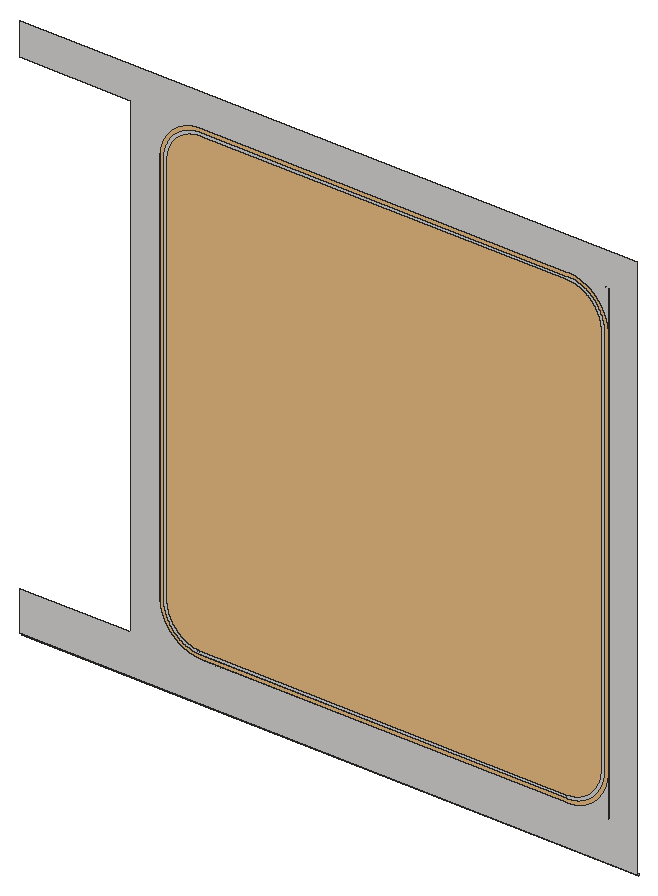
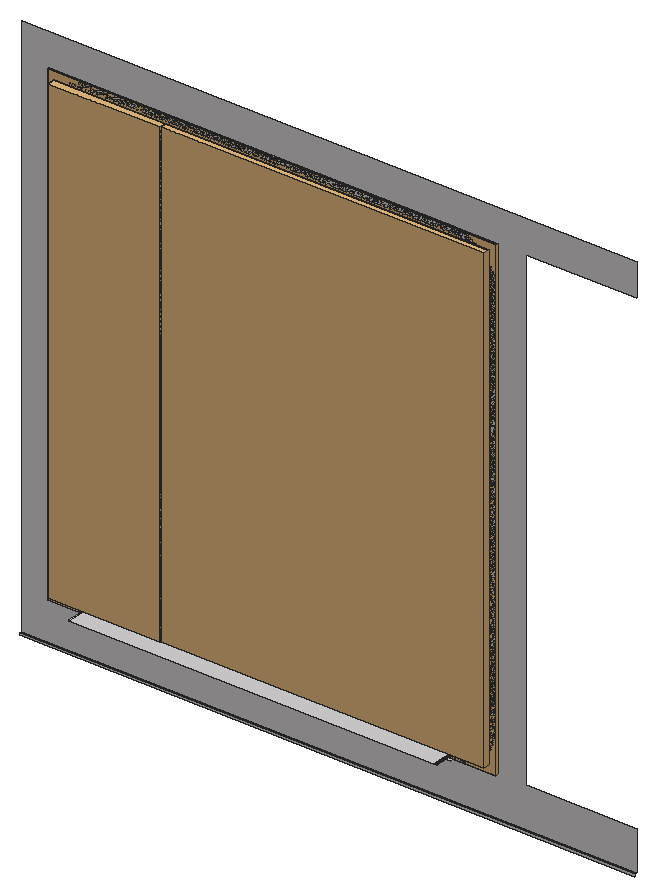
# SketchUp Ruby script. Lengths in inches.
U = 1.inch
M = Sketchup.active_model
def pt(a) = Geom::Point3d.new(a.map { |v| v * U })
def face(e, loops, mat)
  f = e.add_face(loops[0].map { |a| pt(a) })
  loops[1..].each { |l| e.add_face(l.map { |a| pt(a) }).erase! }
  f.material = f.back_material = mat if mat
  f
end
# faces: each face lists its corners as indices into pts; further lists are holes
def faces(e, pts, list, mat = nil) = list.each { |f| face(e, (f[0].is_a?(Array) ? f : [f]).map { |l| l.map { |i| pts[i] } }, mat) }
# xy, xz, yz: faces in a plane at the given z, y or x. An outline is a flat list of corners, or four numbers for a rectangle; further outlines are holes
def ring(l) = l.size == 4 ? [[l[0], l[1]], [l[2], l[1]], [l[2], l[3]], [l[0], l[3]]] : l.each_slice(2).to_a
def flat(e, list, mat, &to3) = list.each { |f| face(e, (f[0].is_a?(Array) ? f : [f]).map { |l| ring(l).map { |u, v| to3.(u, v) } }, mat) }
def xy(e, z, list, mat = nil) = flat(e, list, mat) { |x, y| [x, y, z] }
def xz(e, y, list, mat = nil) = flat(e, list, mat) { |x, z| [x, y, z] }
def yz(e, x, list, mat = nil) = flat(e, list, mat) { |y, z| [x, y, z] }
def lines(e, pts, list) = list.each { |a, b| e.add_line(pt(pts[a]), pt(pts[b])) }
# prism: a flat outline (further loops are holes) pulled along v
def prism(e, loops, v, mat = nil)
  f = face(e, loops, mat); d = Geom::Vector3d.new(v.map { |x| x * U })
  f.pushpull(f.normal.samedirection?(d) ? d.length : -d.length)
end
def box(e, o, s, mat = nil) = prism(e, [[o, [o[0] + s[0], o[1], o[2]], [o[0] + s[0], o[1] + s[1], o[2]], [o[0], o[1] + s[1], o[2]]]], [0, 0, s[2]], mat)
def at(x, y, z, deg = 0) = Geom::Transformation.translation(pt([x, y, z])) * Geom::Transformation.rotation(ORIGIN, Z_AXIS, deg.degrees)
def axes(o, x, y, z) = Geom::Transformation.new([*x, 0, *y, 0, *z, 0, *pt(o).to_a, 1])
def part(name) = M.definitions.add(name)
# library, detail: a bought-in or finely detailed component or shape, given as its bounding box
def library(name, o, s) = part(name).tap { |d| box(d.entities, o, s) }
def detail(e, o, s) = box(e.add_group.entities, o, s)
def put(e, d, t, mat = nil) = e.add_instance(d, t).tap { |i| i.material = mat if mat }
def group(e, t, mat = nil) = e.add_group.tap { |g| g.transformation = t; g.material = mat if mat }.entities
root = M.entities
M.materials.add("Outer Light - 1").color = [251, 216, 141]
M.materials.add("T METAL").color = [42, 41, 39]
M.materials.add("[Quartz Light Brown]").color = [215, 212, 212]
M.materials.add("[Wood Veneer 01]").color = [93, 57, 34]
c1 = library("Group\#11",[0,-3,0],[138.5,2.5,198])
c2 = library("Group\#6",[0,0,0],[192.5,1,204])
c3 = library("Group\#9",[0,0,0],[48,3,198])
xy(root,150,[[293.26,143,293.5,144.25],[293.5,143,450,144.25],[450,143,450.24,144.25],[293.5,144.25,450,146]],"[Quartz Light Brown]")
xy(root,150.01,[[292.79,143,293.03,144.25]],"[Quartz Light Brown]")
xy(root,152,[[293.29,143,293.5,144.25],[293.5,143,450,144.25],[450,143,450.21,144.25]],"[Quartz Light Brown]")
xy(root,152.01,[[292.87,143,293.08,144.25]],"[Quartz Light Brown]")
xy(root,153,[[293.3,143,293.5,155],[293.5,143,450,155],[450,143,450.2,155]],"[Quartz Light Brown]")
xy(root,153.01,[[292.91,143,293.11,155]],"[Quartz Light Brown]")
xz(root,143,[[[216,133,480,133,480,368,216,368,216,354,263.5,354,263.5,150,216,150],[293.26,150,293.03,150.01,292.79,150.01,292.56,150.02,292.32,150.04,292.09,150.06,291.85,150.08,291.62,150.1,291.38,150.125,291.15,150.15,290.92,150.1875,290.68,150.22,290.22,150.3,289.99,150.35,289.76,150.39,289.53,150.44,289.3,150.5,289.07,150.55,288.84,150.61,288.61,150.68,288.39,150.74,288.16,150.81,287.9375,150.88,287.71,150.96,287.49,151.03,287.27,151.11,287.05,151.2,286.83,151.28,286.39,151.46,286.18,151.56,285.96,151.65,285.75,151.75,285.54,151.86,285.33,151.96,284.91,152.18,284.7,152.3,284.5,152.41,284.1,152.65,283.89,152.78,283.7,152.9,283.5,153.03,283.3,153.17,283.11,153.3,282.92,153.4375,282.73,153.58,282.54,153.72,282.36,153.86,282.17,154.01,281.99,154.16,281.81,154.3125,281.63,154.47,281.46,154.625,281.28,154.78,281.11,154.94,280.94,155.11,280.77,155.27,280.61,155.44,280.44,155.61,280.28,155.78,280.125,155.96,279.97,156.13,279.8125,156.31,279.66,156.49,279.51,156.67,279.36,156.86,279.22,157.04,279.08,157.23,278.9375,157.42,278.8,157.61,278.67,157.8,278.53,158,278.4,158.2,278.28,158.39,278.15,158.6,277.91,159,277.8,159.2,277.68,159.41,277.46,159.83,277.36,160.04,277.25,160.25,277.15,160.46,277.06,160.68,276.96,160.89,276.78,161.33,276.7,161.55,276.61,161.77,276.53,161.99,276.46,162.21,276.38,162.4375,276.31,162.66,276.24,162.89,276.18,163.11,276.11,163.34,276.05,163.57,276,163.8,275.94,164.03,275.89,164.26,275.85,164.49,275.8,164.72,275.72,165.18,275.6875,165.42,275.65,165.65,275.625,165.88,275.6,166.12,275.58,166.35,275.56,166.59,275.54,166.82,275.52,167.06,275.51,167.29,275.51,167.53,275.5,167.76,275.5,336.24,275.51,336.47,275.51,336.71,275.52,336.94,275.54,337.18,275.56,337.41,275.58,337.65,275.6,337.88,275.625,338.12,275.65,338.35,275.6875,338.58,275.72,338.82,275.8,339.28,275.85,339.51,275.89,339.74,275.94,339.97,276,340.2,276.05,340.43,276.11,340.66,276.18,340.89,276.24,341.11,276.31,341.34,276.38,341.5625,276.46,341.79,276.53,342.01,276.61,342.23,276.7,342.45,276.78,342.67,276.96,343.11,277.06,343.32,277.15,343.54,277.25,343.75,277.36,343.96,277.46,344.17,277.68,344.59,277.8,344.8,277.91,345,278.15,345.4,278.28,345.61,278.4,345.8,278.53,346,278.67,346.2,278.8,346.39,278.9375,346.58,279.08,346.77,279.22,346.96,279.36,347.14,279.51,347.33,279.66,347.51,279.8125,347.69,279.97,347.87,280.125,348.04,280.28,348.22,280.44,348.39,280.61,348.56,280.77,348.73,280.94,348.89,281.11,349.06,281.28,349.22,281.46,349.375,281.63,349.53,281.81,349.6875,281.99,349.84,282.17,349.99,282.36,350.14,282.54,350.28,282.73,350.42,282.92,350.5625,283.11,350.7,283.3,350.83,283.5,350.97,283.7,351.1,283.89,351.22,284.1,351.35,284.5,351.59,284.7,351.7,284.91,351.82,285.33,352.04,285.54,352.14,285.75,352.25,285.96,352.35,286.18,352.44,286.39,352.54,286.83,352.72,287.05,352.8,287.27,352.89,287.49,352.97,287.71,353.04,287.9375,353.12,288.16,353.19,288.39,353.26,288.61,353.32,288.84,353.39,289.07,353.45,289.3,353.5,289.53,353.56,289.76,353.61,289.99,353.65,290.22,353.7,290.68,353.78,290.92,353.8125,291.15,353.85,291.38,353.875,291.62,353.9,291.85,353.92,292.09,353.94,292.32,353.96,292.56,353.98,292.79,353.99,293.03,353.99,293.26,354,450.24,354,450.47,353.99,450.71,353.99,450.94,353.98,451.18,353.96,451.41,353.94,451.65,353.92,451.88,353.9,452.12,353.875,452.35,353.85,452.58,353.8125,452.82,353.78,453.28,353.7,453.51,353.65,453.74,353.61,453.97,353.56,454.2,353.5,454.43,353.45,454.66,353.39,454.89,353.32,455.11,353.26,455.34,353.19,455.5625,353.12,455.79,353.04,456.01,352.97,456.23,352.89,456.45,352.8,456.67,352.72,457.11,352.54,457.32,352.44,457.54,352.35,457.75,352.25,457.96,352.14,458.17,352.04,458.59,351.82,458.8,351.7,459,351.59,459.4,351.35,459.61,351.22,459.8,351.1,460,350.97,460.2,350.83,460.39,350.7,460.58,350.5625,460.77,350.42,460.96,350.28,461.14,350.14,461.33,349.99,461.51,349.84,461.69,349.6875,461.87,349.53,462.04,349.375,462.22,349.22,462.39,349.06,462.56,348.89,462.73,348.73,462.89,348.56,463.06,348.39,463.22,348.22,463.375,348.04,463.53,347.87,463.6875,347.69,463.84,347.51,463.99,347.33,464.14,347.14,464.28,346.96,464.42,346.77,464.5625,346.58,464.7,346.39,464.83,346.2,464.97,346,465.1,345.8,465.22,345.61,465.35,345.4,465.59,345,465.7,344.8,465.82,344.59,466.04,344.17,466.14,343.96,466.25,343.75,466.35,343.54,466.44,343.32,466.54,343.11,466.72,342.67,466.8,342.45,466.89,342.23,466.97,342.01,467.04,341.79,467.12,341.5625,467.19,341.34,467.26,341.11,467.32,340.89,467.39,340.66,467.45,340.43,467.5,340.2,467.56,339.97,467.61,339.74,467.65,339.51,467.7,339.28,467.78,338.82,467.8125,338.58,467.85,338.35,467.875,338.12,467.9,337.88,467.92,337.65,467.94,337.41,467.96,337.18,467.98,336.94,467.99,336.71,467.99,336.47,468,336.24,468,167.76,467.99,167.53,467.99,167.29,467.98,167.06,467.96,166.82,467.94,166.59,467.92,166.35,467.9,166.12,467.875,165.88,467.85,165.65,467.8125,165.42,467.78,165.18,467.7,164.72,467.65,164.49,467.61,164.26,467.56,164.03,467.5,163.8,467.45,163.57,467.39,163.34,467.32,163.11,467.26,162.89,467.19,162.66,467.12,162.4375,467.04,162.21,466.97,161.99,466.89,161.77,466.8,161.55,466.72,161.33,466.54,160.89,466.44,160.68,466.35,160.46,466.25,160.25,466.14,160.04,466.04,159.83,465.82,159.41,465.7,159.2,465.59,159,465.35,158.6,465.22,158.39,465.1,158.2,464.97,158,464.83,157.8,464.7,157.61,464.5625,157.42,464.42,157.23,464.28,157.04,464.14,156.86,463.99,156.67,463.84,156.49,463.6875,156.31,463.53,156.13,463.375,155.96,463.22,155.78,463.06,155.61,462.89,155.44,462.73,155.27,462.56,155.11,462.39,154.94,462.22,154.78,462.04,154.625,461.87,154.47,461.69,154.3125,461.51,154.16,461.33,154.01,461.14,153.86,460.96,153.72,460.77,153.58,460.58,153.4375,460.39,153.3,460.2,153.17,460,153.03,459.8,152.9,459.61,152.78,459.4,152.65,459,152.41,458.8,152.3,458.59,152.18,458.17,151.96,457.96,151.86,457.75,151.75,457.54,151.65,457.32,151.56,457.11,151.46,456.67,151.28,456.45,151.2,456.23,151.11,456.01,151.03,455.79,150.96,455.5625,150.88,455.34,150.81,455.11,150.74,454.89,150.68,454.66,150.61,454.43,150.55,454.2,150.5,453.97,150.44,453.74,150.39,453.51,150.35,453.28,150.3,452.82,150.22,452.58,150.1875,452.35,150.15,452.12,150.125,451.88,150.1,451.65,150.08,451.41,150.06,451.18,150.04,450.94,150.02,450.71,150.01,450.47,150.01,450.24,150]],[[293.29,152,450.21,152,450.42,152.01,450.63,152.01,451.05,152.03,451.26,152.05,451.46,152.07,451.88,152.11,452.3,152.17,452.5,152.2,452.71,152.23,452.92,152.27,453.12,152.31,453.33,152.35,453.53,152.39,453.74,152.44,453.9375,152.49,454.14,152.55,454.34,152.6,454.94,152.78,455.54,152.99,455.73,153.0625,455.93,153.14,456.12,153.22,456.32,153.3,456.51,153.38,457.08,153.65,457.26,153.74,457.45,153.84,457.63,153.9375,457.82,154.04,458,154.14,458.54,154.47,458.71,154.58,458.89,154.7,459.0625,154.8125,459.23,154.93,459.4,155.06,459.57,155.18,459.74,155.31,459.91,155.43,460.07,155.57,460.39,155.83,460.71,156.11,461.01,156.39,461.16,156.54,461.3125,156.6875,461.46,156.84,461.61,156.99,461.89,157.29,462.17,157.61,462.43,157.93,462.57,158.09,462.69,158.26,462.82,158.43,462.94,158.6,463.07,158.77,463.1875,158.9375,463.3,159.11,463.42,159.29,463.53,159.46,463.86,160,463.96,160.18,464.0625,160.37,464.16,160.55,464.26,160.74,464.35,160.92,464.62,161.49,464.7,161.68,464.78,161.88,464.86,162.07,464.9375,162.27,465.01,162.46,465.22,163.06,465.4,163.66,465.45,163.86,465.51,164.0625,465.56,164.26,465.61,164.47,465.65,164.67,465.69,164.88,465.73,165.08,465.77,165.29,465.8,165.5,465.83,165.7,465.89,166.12,465.93,166.54,465.95,166.74,465.97,166.95,465.99,167.37,465.99,167.58,466,167.79,466,336.21,465.99,336.42,465.99,336.63,465.97,337.05,465.95,337.26,465.93,337.46,465.89,337.88,465.83,338.3,465.8,338.5,465.77,338.71,465.73,338.92,465.69,339.12,465.65,339.33,465.61,339.53,465.56,339.74,465.51,339.9375,465.45,340.14,465.4,340.34,465.22,340.94,465.01,341.54,464.9375,341.73,464.86,341.93,464.78,342.12,464.7,342.32,464.62,342.51,464.35,343.08,464.26,343.26,464.16,343.45,464.0625,343.63,463.96,343.82,463.86,344,463.53,344.54,463.42,344.71,463.3,344.89,463.1875,345.0625,463.07,345.23,462.94,345.4,462.82,345.57,462.69,345.74,462.57,345.91,462.43,346.07,462.17,346.39,461.89,346.71,461.61,347.01,461.46,347.16,461.3125,347.3125,461.16,347.46,461.01,347.61,460.71,347.89,460.39,348.17,460.07,348.43,459.91,348.57,459.74,348.69,459.57,348.82,459.4,348.94,459.23,349.07,459.0625,349.1875,458.89,349.3,458.71,349.42,458.54,349.53,458,349.86,457.82,349.96,457.63,350.0625,457.45,350.16,457.26,350.26,457.08,350.35,456.51,350.62,456.32,350.7,456.12,350.78,455.93,350.86,455.73,350.9375,455.54,351.01,454.94,351.22,454.34,351.4,454.14,351.45,453.9375,351.51,453.74,351.56,453.53,351.61,453.33,351.65,453.12,351.69,452.92,351.73,452.71,351.77,452.5,351.8,452.3,351.83,451.88,351.89,451.46,351.93,451.26,351.95,451.05,351.97,450.63,351.99,450.42,351.99,450.21,352,293.29,352,293.08,351.99,292.87,351.99,292.45,351.97,292.24,351.95,292.04,351.93,291.62,351.89,291.2,351.83,291,351.8,290.79,351.77,290.58,351.73,290.38,351.69,290.17,351.65,289.97,351.61,289.76,351.56,289.5625,351.51,289.36,351.45,289.16,351.4,288.56,351.22,287.96,351.01,287.77,350.9375,287.57,350.86,287.38,350.78,287.18,350.7,286.99,350.62,286.42,350.35,286.24,350.26,286.05,350.16,285.87,350.0625,285.68,349.96,285.5,349.86,284.96,349.53,284.79,349.42,284.61,349.3,284.4375,349.1875,284.27,349.07,284.1,348.94,283.93,348.82,283.76,348.69,283.59,348.57,283.43,348.43,283.11,348.17,282.79,347.89,282.49,347.61,282.34,347.46,282.1875,347.3125,282.04,347.16,281.89,347.01,281.61,346.71,281.33,346.39,281.07,346.07,280.93,345.91,280.81,345.74,280.68,345.57,280.56,345.4,280.43,345.23,280.3125,345.0625,280.2,344.89,280.08,344.71,279.97,344.54,279.64,344,279.54,343.82,279.4375,343.63,279.34,343.45,279.24,343.26,279.15,343.08,278.88,342.51,278.8,342.32,278.72,342.12,278.64,341.93,278.5625,341.73,278.49,341.54,278.28,340.94,278.1,340.34,278.05,340.14,277.99,339.9375,277.94,339.74,277.89,339.53,277.85,339.33,277.81,339.12,277.77,338.92,277.73,338.71,277.7,338.5,277.67,338.3,277.61,337.88,277.57,337.46,277.55,337.26,277.53,337.05,277.51,336.63,277.51,336.42,277.5,336.21,277.5,167.79,277.51,167.58,277.51,167.37,277.53,166.95,277.55,166.74,277.57,166.54,277.61,166.12,277.67,165.7,277.7,165.5,277.73,165.29,277.77,165.08,277.81,164.88,277.85,164.67,277.89,164.47,277.94,164.26,277.99,164.0625,278.05,163.86,278.1,163.66,278.28,163.06,278.49,162.46,278.5625,162.27,278.64,162.07,278.72,161.88,278.8,161.68,278.88,161.49,279.15,160.92,279.24,160.74,279.34,160.55,279.4375,160.37,279.54,160.18,279.64,160,279.97,159.46,280.08,159.29,280.2,159.11,280.3125,158.9375,280.43,158.77,280.56,158.6,280.68,158.43,280.81,158.26,280.93,158.09,281.07,157.93,281.33,157.61,281.61,157.29,281.89,156.99,282.04,156.84,282.1875,156.6875,282.34,156.54,282.49,156.39,282.79,156.11,283.11,155.83,283.43,155.57,283.59,155.43,283.76,155.31,283.93,155.18,284.1,155.06,284.27,154.93,284.4375,154.8125,284.61,154.7,284.79,154.58,284.96,154.47,285.5,154.14,285.68,154.04,285.87,153.9375,286.05,153.84,286.24,153.74,286.42,153.65,286.99,153.38,287.18,153.3,287.38,153.22,287.57,153.14,287.77,153.0625,287.96,152.99,288.56,152.78,289.16,152.6,289.36,152.55,289.5625,152.49,289.76,152.44,289.97,152.39,290.17,152.35,290.38,152.31,290.58,152.27,290.79,152.23,291,152.2,291.2,152.17,291.62,152.11,292.04,152.07,292.24,152.05,292.45,152.03,292.87,152.01,293.08,152.01],[293.3,153,293.11,153.01,292.91,153.01,292.71,153.02,292.52,153.03,292.32,153.05,292.13,153.0625,291.93,153.08,291.74,153.1,291.54,153.13,291.35,153.16,291.15,153.18,290.96,153.22,290.77,153.25,290.57,153.29,290,153.41,289.62,153.51,289.43,153.5625,289.24,153.62,289.05,153.67,288.86,153.73,288.68,153.8,288.49,153.86,288.31,153.93,287.94,154.07,287.76,154.14,287.04,154.46,286.87,154.55,286.69,154.63,286.52,154.73,286.34,154.82,286.17,154.91,285.66,155.21,285.5,155.3125,285.33,155.42,285.17,155.53,285,155.64,284.68,155.86,284.53,155.98,284.21,156.22,284.06,156.34,283.91,156.47,283.76,156.59,283.46,156.85,283.32,156.99,283.17,157.12,283.03,157.26,282.89,157.39,282.76,157.53,282.62,157.67,282.49,157.82,282.35,157.96,282.09,158.26,281.97,158.41,281.84,158.56,281.72,158.71,281.48,159.03,281.36,159.18,281.14,159.5,281.03,159.67,280.92,159.83,280.8125,160,280.71,160.16,280.41,160.67,280.32,160.84,280.23,161.02,280.13,161.19,280.05,161.37,279.96,161.54,279.64,162.26,279.57,162.44,279.43,162.81,279.36,162.99,279.3,163.18,279.23,163.36,279.17,163.55,279.12,163.74,279.0625,163.93,279.01,164.12,278.91,164.5,278.79,165.07,278.75,165.27,278.72,165.46,278.68,165.65,278.66,165.85,278.63,166.04,278.6,166.24,278.58,166.43,278.5625,166.63,278.55,166.82,278.53,167.02,278.52,167.21,278.51,167.41,278.51,167.61,278.5,167.8,278.5,336.2,278.51,336.39,278.51,336.59,278.52,336.79,278.53,336.98,278.55,337.18,278.5625,337.37,278.58,337.57,278.6,337.76,278.63,337.96,278.66,338.15,278.68,338.35,278.72,338.54,278.75,338.73,278.79,338.93,278.91,339.5,279.01,339.88,279.0625,340.07,279.12,340.26,279.17,340.45,279.23,340.64,279.3,340.82,279.36,341.01,279.43,341.19,279.57,341.56,279.64,341.74,279.96,342.46,280.05,342.63,280.13,342.81,280.23,342.98,280.32,343.16,280.41,343.33,280.71,343.84,280.8125,344,280.92,344.17,281.03,344.33,281.14,344.5,281.36,344.82,281.48,344.97,281.72,345.29,281.84,345.44,281.97,345.59,282.09,345.74,282.35,346.04,282.49,346.18,282.62,346.33,282.76,346.47,282.89,346.61,283.03,346.74,283.17,346.88,283.32,347.01,283.46,347.15,283.76,347.41,283.91,347.53,284.06,347.66,284.21,347.78,284.53,348.02,284.68,348.14,285,348.36,285.17,348.47,285.33,348.58,285.5,348.6875,285.66,348.79,286.17,349.09,286.34,349.18,286.52,349.27,286.69,349.37,286.87,349.45,287.04,349.54,287.76,349.86,287.94,349.93,288.31,350.07,288.49,350.14,288.68,350.2,288.86,350.27,289.05,350.33,289.24,350.38,289.43,350.4375,289.62,350.49,290,350.59,290.57,350.71,290.77,350.75,290.96,350.78,291.15,350.82,291.35,350.84,291.54,350.87,291.74,350.9,291.93,350.92,292.13,350.9375,292.32,350.95,292.52,350.97,292.71,350.98,292.91,350.99,293.11,350.99,293.3,351,450.2,351,450.39,350.99,450.59,350.99,450.79,350.98,450.98,350.97,451.18,350.95,451.37,350.9375,451.57,350.92,451.76,350.9,451.96,350.87,452.15,350.84,452.35,350.82,452.54,350.78,452.73,350.75,452.93,350.71,453.5,350.59,453.88,350.49,454.07,350.4375,454.26,350.38,454.45,350.33,454.64,350.27,454.82,350.2,455.01,350.14,455.19,350.07,455.56,349.93,455.74,349.86,456.46,349.54,456.63,349.45,456.81,349.37,456.98,349.27,457.16,349.18,457.33,349.09,457.84,348.79,458,348.6875,458.17,348.58,458.33,348.47,458.5,348.36,458.82,348.14,458.97,348.02,459.29,347.78,459.44,347.66,459.59,347.53,459.74,347.41,460.04,347.15,460.18,347.01,460.33,346.88,460.47,346.74,460.61,346.61,460.74,346.47,460.88,346.33,461.01,346.18,461.15,346.04,461.41,345.74,461.53,345.59,461.66,345.44,461.78,345.29,462.02,344.97,462.14,344.82,462.36,344.5,462.47,344.33,462.58,344.17,462.6875,344,462.79,343.84,463.09,343.33,463.18,343.16,463.27,342.98,463.37,342.81,463.45,342.63,463.54,342.46,463.86,341.74,463.93,341.56,464.07,341.19,464.14,341.01,464.2,340.82,464.27,340.64,464.33,340.45,464.38,340.26,464.4375,340.07,464.49,339.88,464.59,339.5,464.71,338.93,464.75,338.73,464.78,338.54,464.82,338.35,464.84,338.15,464.87,337.96,464.9,337.76,464.92,337.57,464.9375,337.37,464.95,337.18,464.97,336.98,464.98,336.79,464.99,336.59,464.99,336.39,465,336.2,465,167.8,464.99,167.61,464.99,167.41,464.98,167.21,464.97,167.02,464.95,166.82,464.9375,166.63,464.92,166.43,464.9,166.24,464.87,166.04,464.84,165.85,464.82,165.65,464.78,165.46,464.75,165.27,464.71,165.07,464.59,164.5,464.49,164.12,464.4375,163.93,464.38,163.74,464.33,163.55,464.27,163.36,464.2,163.18,464.14,162.99,464.07,162.81,463.93,162.44,463.86,162.26,463.54,161.54,463.45,161.37,463.37,161.19,463.27,161.02,463.18,160.84,463.09,160.67,462.79,160.16,462.6875,160,462.58,159.83,462.47,159.67,462.36,159.5,462.14,159.18,462.02,159.03,461.78,158.71,461.66,158.56,461.53,158.41,461.41,158.26,461.15,157.96,461.01,157.82,460.88,157.67,460.74,157.53,460.61,157.39,460.47,157.26,460.33,157.12,460.18,156.99,460.04,156.85,459.74,156.59,459.59,156.47,459.44,156.34,459.29,156.22,458.97,155.98,458.82,155.86,458.5,155.64,458.33,155.53,458.17,155.42,458,155.3125,457.84,155.21,457.33,154.91,457.16,154.82,456.98,154.73,456.81,154.63,456.63,154.55,456.46,154.46,455.74,154.14,455.56,154.07,455.19,153.93,455.01,153.86,454.82,153.8,454.64,153.73,454.45,153.67,454.26,153.62,454.07,153.5625,453.88,153.51,453.5,153.41,452.93,153.29,452.73,153.25,452.54,153.22,452.35,153.18,452.15,153.16,451.96,153.13,451.76,153.1,451.57,153.08,451.37,153.0625,451.18,153.05,450.98,153.03,450.79,153.02,450.59,153.01,450.39,153.01,450.2,153]]],"[Quartz Light Brown]")
xz(root,144,[[216,132,480,133]],"[Quartz Light Brown]")
xz(root,144.25,[[[293.26,150,450.24,150,450.47,150.01,450.71,150.01,450.94,150.02,451.18,150.04,451.41,150.06,451.65,150.08,451.88,150.1,452.12,150.125,452.35,150.15,452.58,150.1875,452.82,150.22,453.28,150.3,453.51,150.35,453.74,150.39,453.97,150.44,454.2,150.5,454.43,150.55,454.66,150.61,454.89,150.68,455.11,150.74,455.34,150.81,455.5625,150.88,455.79,150.96,456.01,151.03,456.23,151.11,456.45,151.2,456.67,151.28,457.11,151.46,457.32,151.56,457.54,151.65,457.75,151.75,457.96,151.86,458.17,151.96,458.59,152.18,458.8,152.3,459,152.41,459.4,152.65,459.61,152.78,459.8,152.9,460,153.03,460.2,153.17,460.39,153.3,460.58,153.4375,460.77,153.58,460.96,153.72,461.14,153.86,461.33,154.01,461.51,154.16,461.69,154.3125,461.87,154.47,462.04,154.625,462.22,154.78,462.39,154.94,462.56,155.11,462.73,155.27,462.89,155.44,463.06,155.61,463.22,155.78,463.375,155.96,463.53,156.13,463.6875,156.31,463.84,156.49,463.99,156.67,464.14,156.86,464.28,157.04,464.42,157.23,464.5625,157.42,464.7,157.61,464.83,157.8,464.97,158,465.1,158.2,465.22,158.39,465.35,158.6,465.59,159,465.7,159.2,465.82,159.41,466.04,159.83,466.14,160.04,466.25,160.25,466.35,160.46,466.44,160.68,466.54,160.89,466.72,161.33,466.8,161.55,466.89,161.77,466.97,161.99,467.04,162.21,467.12,162.4375,467.19,162.66,467.26,162.89,467.32,163.11,467.39,163.34,467.45,163.57,467.5,163.8,467.56,164.03,467.61,164.26,467.65,164.49,467.7,164.72,467.78,165.18,467.8125,165.42,467.85,165.65,467.875,165.88,467.9,166.12,467.92,166.35,467.94,166.59,467.96,166.82,467.98,167.06,467.99,167.29,467.99,167.53,468,167.76,468,336.24,467.99,336.47,467.99,336.71,467.98,336.94,467.96,337.18,467.94,337.41,467.92,337.65,467.9,337.88,467.875,338.12,467.85,338.35,467.8125,338.58,467.78,338.82,467.7,339.28,467.65,339.51,467.61,339.74,467.56,339.97,467.5,340.2,467.45,340.43,467.39,340.66,467.32,340.89,467.26,341.11,467.19,341.34,467.12,341.5625,467.04,341.79,466.97,342.01,466.89,342.23,466.8,342.45,466.72,342.67,466.54,343.11,466.44,343.32,466.35,343.54,466.25,343.75,466.14,343.96,466.04,344.17,465.82,344.59,465.7,344.8,465.59,345,465.35,345.4,465.22,345.61,465.1,345.8,464.97,346,464.83,346.2,464.7,346.39,464.5625,346.58,464.42,346.77,464.28,346.96,464.14,347.14,463.99,347.33,463.84,347.51,463.6875,347.69,463.53,347.87,463.375,348.04,463.22,348.22,463.06,348.39,462.89,348.56,462.73,348.73,462.56,348.89,462.39,349.06,462.22,349.22,462.04,349.375,461.87,349.53,461.69,349.6875,461.51,349.84,461.33,349.99,461.14,350.14,460.96,350.28,460.77,350.42,460.58,350.5625,460.39,350.7,460.2,350.83,460,350.97,459.8,351.1,459.61,351.22,459.4,351.35,459,351.59,458.8,351.7,458.59,351.82,458.17,352.04,457.96,352.14,457.75,352.25,457.54,352.35,457.32,352.44,457.11,352.54,456.67,352.72,456.45,352.8,456.23,352.89,456.01,352.97,455.79,353.04,455.5625,353.12,455.34,353.19,455.11,353.26,454.89,353.32,454.66,353.39,454.43,353.45,454.2,353.5,453.97,353.56,453.74,353.61,453.51,353.65,453.28,353.7,452.82,353.78,452.58,353.8125,452.35,353.85,452.12,353.875,451.88,353.9,451.65,353.92,451.41,353.94,451.18,353.96,450.94,353.98,450.71,353.99,450.47,353.99,450.24,354,293.26,354,293.03,353.99,292.79,353.99,292.56,353.98,292.32,353.96,292.09,353.94,291.85,353.92,291.62,353.9,291.38,353.875,291.15,353.85,290.92,353.8125,290.68,353.78,290.22,353.7,289.99,353.65,289.76,353.61,289.53,353.56,289.3,353.5,289.07,353.45,288.84,353.39,288.61,353.32,288.39,353.26,288.16,353.19,287.9375,353.12,287.71,353.04,287.49,352.97,287.27,352.89,287.05,352.8,286.83,352.72,286.39,352.54,286.18,352.44,285.96,352.35,285.75,352.25,285.54,352.14,285.33,352.04,284.91,351.82,284.7,351.7,284.5,351.59,284.1,351.35,283.89,351.22,283.7,351.1,283.5,350.97,283.3,350.83,283.11,350.7,282.92,350.5625,282.73,350.42,282.54,350.28,282.36,350.14,282.17,349.99,281.99,349.84,281.81,349.6875,281.63,349.53,281.46,349.375,281.28,349.22,281.11,349.06,280.94,348.89,280.77,348.73,280.61,348.56,280.44,348.39,280.28,348.22,280.125,348.04,279.97,347.87,279.8125,347.69,279.66,347.51,279.51,347.33,279.36,347.14,279.22,346.96,279.08,346.77,278.9375,346.58,278.8,346.39,278.67,346.2,278.53,346,278.4,345.8,278.28,345.61,278.15,345.4,277.91,345,277.8,344.8,277.68,344.59,277.46,344.17,277.36,343.96,277.25,343.75,277.15,343.54,277.06,343.32,276.96,343.11,276.78,342.67,276.7,342.45,276.61,342.23,276.53,342.01,276.46,341.79,276.38,341.5625,276.31,341.34,276.24,341.11,276.18,340.89,276.11,340.66,276.05,340.43,276,340.2,275.94,339.97,275.89,339.74,275.85,339.51,275.8,339.28,275.72,338.82,275.6875,338.58,275.65,338.35,275.625,338.12,275.6,337.88,275.58,337.65,275.56,337.41,275.54,337.18,275.52,336.94,275.51,336.71,275.51,336.47,275.5,336.24,275.5,167.76,275.51,167.53,275.51,167.29,275.52,167.06,275.54,166.82,275.56,166.59,275.58,166.35,275.6,166.12,275.625,165.88,275.65,165.65,275.6875,165.42,275.72,165.18,275.8,164.72,275.85,164.49,275.89,164.26,275.94,164.03,276,163.8,276.05,163.57,276.11,163.34,276.18,163.11,276.24,162.89,276.31,162.66,276.38,162.4375,276.46,162.21,276.53,161.99,276.61,161.77,276.7,161.55,276.78,161.33,276.96,160.89,277.06,160.68,277.15,160.46,277.25,160.25,277.36,160.04,277.46,159.83,277.68,159.41,277.8,159.2,277.91,159,278.15,158.6,278.28,158.39,278.4,158.2,278.53,158,278.67,157.8,278.8,157.61,278.9375,157.42,279.08,157.23,279.22,157.04,279.36,156.86,279.51,156.67,279.66,156.49,279.8125,156.31,279.97,156.13,280.125,155.96,280.28,155.78,280.44,155.61,280.61,155.44,280.77,155.27,280.94,155.11,281.11,154.94,281.28,154.78,281.46,154.625,281.63,154.47,281.81,154.3125,281.99,154.16,282.17,154.01,282.36,153.86,282.54,153.72,282.73,153.58,282.92,153.4375,283.11,153.3,283.3,153.17,283.5,153.03,283.7,152.9,283.89,152.78,284.1,152.65,284.5,152.41,284.7,152.3,284.91,152.18,285.33,151.96,285.54,151.86,285.75,151.75,285.96,151.65,286.18,151.56,286.39,151.46,286.83,151.28,287.05,151.2,287.27,151.11,287.49,151.03,287.71,150.96,287.9375,150.88,288.16,150.81,288.39,150.74,288.61,150.68,288.84,150.61,289.07,150.55,289.3,150.5,289.53,150.44,289.76,150.39,289.99,150.35,290.22,150.3,290.68,150.22,290.92,150.1875,291.15,150.15,291.38,150.125,291.62,150.1,291.85,150.08,292.09,150.06,292.32,150.04,292.56,150.02,292.79,150.01,293.03,150.01],[293.29,152,293.08,152.01,292.87,152.01,292.45,152.03,292.24,152.05,292.04,152.07,291.62,152.11,291.2,152.17,291,152.2,290.79,152.23,290.58,152.27,290.38,152.31,290.17,152.35,289.97,152.39,289.76,152.44,289.5625,152.49,289.36,152.55,289.16,152.6,288.56,152.78,287.96,152.99,287.77,153.0625,287.57,153.14,287.38,153.22,287.18,153.3,286.99,153.38,286.42,153.65,286.24,153.74,286.05,153.84,285.87,153.9375,285.68,154.04,285.5,154.14,284.96,154.47,284.79,154.58,284.61,154.7,284.4375,154.8125,284.27,154.93,284.1,155.06,283.93,155.18,283.76,155.31,283.59,155.43,283.43,155.57,283.11,155.83,282.79,156.11,282.49,156.39,282.34,156.54,282.1875,156.6875,282.04,156.84,281.89,156.99,281.61,157.29,281.33,157.61,281.07,157.93,280.93,158.09,280.81,158.26,280.68,158.43,280.56,158.6,280.43,158.77,280.3125,158.9375,280.2,159.11,280.08,159.29,279.97,159.46,279.64,160,279.54,160.18,279.4375,160.37,279.34,160.55,279.24,160.74,279.15,160.92,278.88,161.49,278.8,161.68,278.72,161.88,278.64,162.07,278.5625,162.27,278.49,162.46,278.28,163.06,278.1,163.66,278.05,163.86,277.99,164.0625,277.94,164.26,277.89,164.47,277.85,164.67,277.81,164.88,277.77,165.08,277.73,165.29,277.7,165.5,277.67,165.7,277.61,166.12,277.57,166.54,277.55,166.74,277.53,166.95,277.51,167.37,277.51,167.58,277.5,167.79,277.5,336.21,277.51,336.42,277.51,336.63,277.53,337.05,277.55,337.26,277.57,337.46,277.61,337.88,277.67,338.3,277.7,338.5,277.73,338.71,277.77,338.92,277.81,339.12,277.85,339.33,277.89,339.53,277.94,339.74,277.99,339.9375,278.05,340.14,278.1,340.34,278.28,340.94,278.49,341.54,278.5625,341.73,278.64,341.93,278.72,342.12,278.8,342.32,278.88,342.51,279.15,343.08,279.24,343.26,279.34,343.45,279.4375,343.63,279.54,343.82,279.64,344,279.97,344.54,280.08,344.71,280.2,344.89,280.3125,345.0625,280.43,345.23,280.56,345.4,280.68,345.57,280.81,345.74,280.93,345.91,281.07,346.07,281.33,346.39,281.61,346.71,281.89,347.01,282.04,347.16,282.1875,347.3125,282.34,347.46,282.49,347.61,282.79,347.89,283.11,348.17,283.43,348.43,283.59,348.57,283.76,348.69,283.93,348.82,284.1,348.94,284.27,349.07,284.4375,349.1875,284.61,349.3,284.79,349.42,284.96,349.53,285.5,349.86,285.68,349.96,285.87,350.0625,286.05,350.16,286.24,350.26,286.42,350.35,286.99,350.62,287.18,350.7,287.38,350.78,287.57,350.86,287.77,350.9375,287.96,351.01,288.56,351.22,289.16,351.4,289.36,351.45,289.5625,351.51,289.76,351.56,289.97,351.61,290.17,351.65,290.38,351.69,290.58,351.73,290.79,351.77,291,351.8,291.2,351.83,291.62,351.89,292.04,351.93,292.24,351.95,292.45,351.97,292.87,351.99,293.08,351.99,293.29,352,450.21,352,450.42,351.99,450.63,351.99,451.05,351.97,451.26,351.95,451.46,351.93,451.88,351.89,452.3,351.83,452.5,351.8,452.71,351.77,452.92,351.73,453.12,351.69,453.33,351.65,453.53,351.61,453.74,351.56,453.9375,351.51,454.14,351.45,454.34,351.4,454.94,351.22,455.54,351.01,455.73,350.9375,455.93,350.86,456.12,350.78,456.32,350.7,456.51,350.62,457.08,350.35,457.26,350.26,457.45,350.16,457.63,350.0625,457.82,349.96,458,349.86,458.54,349.53,458.71,349.42,458.89,349.3,459.0625,349.1875,459.23,349.07,459.4,348.94,459.57,348.82,459.74,348.69,459.91,348.57,460.07,348.43,460.39,348.17,460.71,347.89,461.01,347.61,461.16,347.46,461.3125,347.3125,461.46,347.16,461.61,347.01,461.89,346.71,462.17,346.39,462.43,346.07,462.57,345.91,462.69,345.74,462.82,345.57,462.94,345.4,463.07,345.23,463.1875,345.0625,463.3,344.89,463.42,344.71,463.53,344.54,463.86,344,463.96,343.82,464.0625,343.63,464.16,343.45,464.26,343.26,464.35,343.08,464.62,342.51,464.7,342.32,464.78,342.12,464.86,341.93,464.9375,341.73,465.01,341.54,465.22,340.94,465.4,340.34,465.45,340.14,465.51,339.9375,465.56,339.74,465.61,339.53,465.65,339.33,465.69,339.12,465.73,338.92,465.77,338.71,465.8,338.5,465.83,338.3,465.89,337.88,465.93,337.46,465.95,337.26,465.97,337.05,465.99,336.63,465.99,336.42,466,336.21,466,167.79,465.99,167.58,465.99,167.37,465.97,166.95,465.95,166.74,465.93,166.54,465.89,166.12,465.83,165.7,465.8,165.5,465.77,165.29,465.73,165.08,465.69,164.88,465.65,164.67,465.61,164.47,465.56,164.26,465.51,164.0625,465.45,163.86,465.4,163.66,465.22,163.06,465.01,162.46,464.9375,162.27,464.86,162.07,464.78,161.88,464.7,161.68,464.62,161.49,464.35,160.92,464.26,160.74,464.16,160.55,464.0625,160.37,463.96,160.18,463.86,160,463.53,159.46,463.42,159.29,463.3,159.11,463.1875,158.9375,463.07,158.77,462.94,158.6,462.82,158.43,462.69,158.26,462.57,158.09,462.43,157.93,462.17,157.61,461.89,157.29,461.61,156.99,461.46,156.84,461.3125,156.6875,461.16,156.54,461.01,156.39,460.71,156.11,460.39,155.83,460.07,155.57,459.91,155.43,459.74,155.31,459.57,155.18,459.4,155.06,459.23,154.93,459.0625,154.8125,458.89,154.7,458.71,154.58,458.54,154.47,458,154.14,457.82,154.04,457.63,153.9375,457.45,153.84,457.26,153.74,457.08,153.65,456.51,153.38,456.32,153.3,456.12,153.22,455.93,153.14,455.73,153.0625,455.54,152.99,454.94,152.78,454.34,152.6,454.14,152.55,453.9375,152.49,453.74,152.44,453.53,152.39,453.33,152.35,453.12,152.31,452.92,152.27,452.71,152.23,452.5,152.2,452.3,152.17,451.88,152.11,451.46,152.07,451.26,152.05,451.05,152.03,450.63,152.01,450.42,152.01,450.21,152]]],"[Quartz Light Brown]")
p = [[292.09,144.25,150.06],[292.09,143,150.06],[292.32,143,150.04],[292.32,144.25,150.04],[292.56,143,150.02],[292.56,144.25,150.02],
  [292.79,143,150.01],[292.79,144.25,150.01],[293.03,144.25,150.01],[293.03,143,150.01],[293.26,143,150],[293.26,144.25,150],
  [292.45,143,152.03],[292.24,143,152.05],[292.24,144.25,152.05],[292.45,144.25,152.03],[292.66,143,152.02],[292.66,144.25,152.02],
  [292.87,143,152.01],[292.87,144.25,152.01],[293.29,143,152],[293.08,143,152.01],[293.08,144.25,152.01],[293.29,144.25,152],
  [450.42,143,152.01],[450.21,143,152],[450.21,144.25,152],[450.42,144.25,152.01],[292.13,143,153.0625],[292.32,143,153.05],
  [292.32,155,153.05],[292.13,155,153.0625],[292.52,143,153.03],[292.52,155,153.03],[292.71,143,153.02],[292.71,155,153.02],
  [292.91,143,153.01],[292.91,155,153.01],[293.11,143,153.01],[293.3,143,153],[293.3,155,153],[293.11,155,153.01],
  [450.2,143,153],[450.39,143,153.01],[450.39,155,153.01],[450.2,155,153]]
faces(root,p,[[0,1,2,3],[3,2,4,5],[5,4,6,7],[8,9,10,11],[12,13,14,15],[16,12,15,17],[18,16,17,19],[20,21,22,23],
  [24,25,26,27],[28,29,30,31],[29,32,33,30],[32,34,35,33],[34,36,37,35],[38,39,40,41],[42,43,44,45]],"[Quartz Light Brown]")
put(root,c1,at(278.5,147.52,153),"T METAL")
put(root,c2,at(275.5,143.25,150),"Outer Light - 1")
put(root,c3,at(417,144.5,153),"[Wood Veneer 01]")
